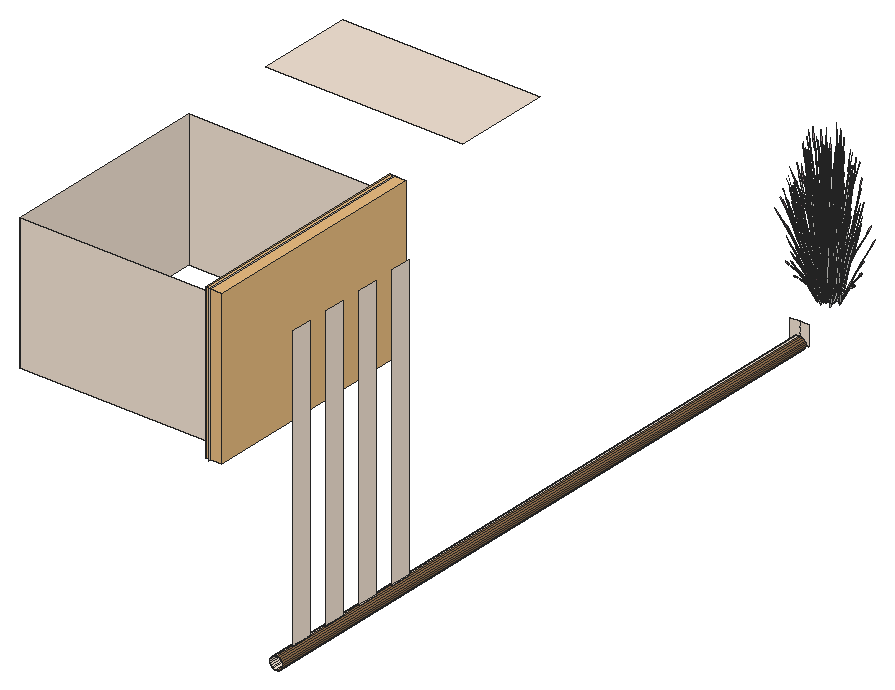
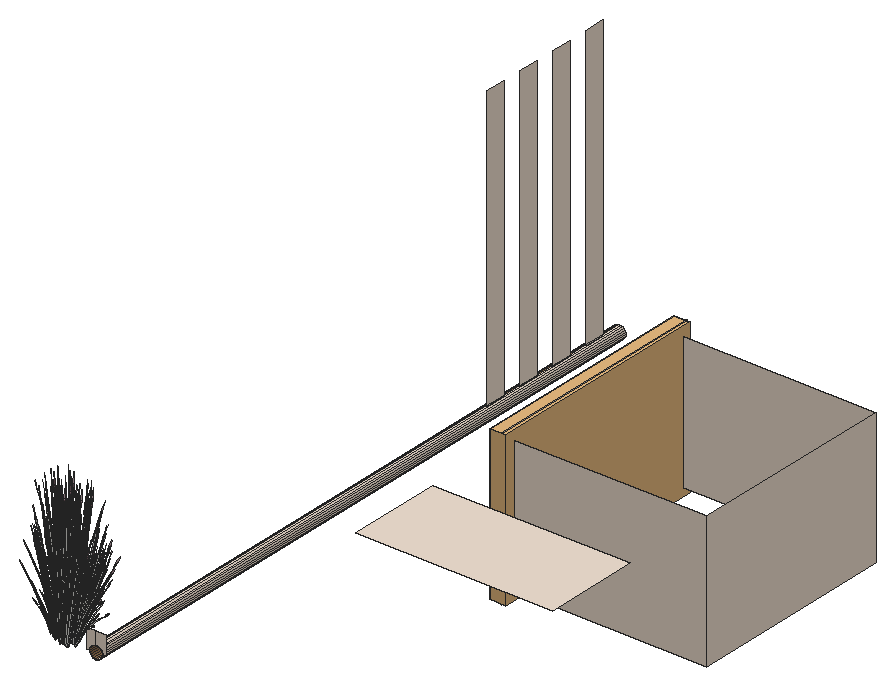
# SketchUp Ruby script. Lengths in inches.
U = 1.inch
M = Sketchup.active_model
def pt(a) = Geom::Point3d.new(a.map { |v| v * U })
def face(e, loops, mat)
  f = e.add_face(loops[0].map { |a| pt(a) })
  loops[1..].each { |l| e.add_face(l.map { |a| pt(a) }).erase! }
  f.material = f.back_material = mat if mat
  f
end
# faces: each face lists its corners as indices into pts; further lists are holes
def faces(e, pts, list, mat = nil) = list.each { |f| face(e, (f[0].is_a?(Array) ? f : [f]).map { |l| l.map { |i| pts[i] } }, mat) }
# xy, xz, yz: faces in a plane at the given z, y or x. An outline is a flat list of corners, or four numbers for a rectangle; further outlines are holes
def ring(l) = l.size == 4 ? [[l[0], l[1]], [l[2], l[1]], [l[2], l[3]], [l[0], l[3]]] : l.each_slice(2).to_a
def flat(e, list, mat, &to3) = list.each { |f| face(e, (f[0].is_a?(Array) ? f : [f]).map { |l| ring(l).map { |u, v| to3.(u, v) } }, mat) }
def xy(e, z, list, mat = nil) = flat(e, list, mat) { |x, y| [x, y, z] }
def xz(e, y, list, mat = nil) = flat(e, list, mat) { |x, z| [x, y, z] }
def yz(e, x, list, mat = nil) = flat(e, list, mat) { |y, z| [x, y, z] }
def lines(e, pts, list) = list.each { |a, b| e.add_line(pt(pts[a]), pt(pts[b])) }
# prism: a flat outline (further loops are holes) pulled along v
def prism(e, loops, v, mat = nil)
  f = face(e, loops, mat); d = Geom::Vector3d.new(v.map { |x| x * U })
  f.pushpull(f.normal.samedirection?(d) ? d.length : -d.length)
end
def box(e, o, s, mat = nil) = prism(e, [[o, [o[0] + s[0], o[1], o[2]], [o[0] + s[0], o[1] + s[1], o[2]], [o[0], o[1] + s[1], o[2]]]], [0, 0, s[2]], mat)
def at(x, y, z, deg = 0) = Geom::Transformation.translation(pt([x, y, z])) * Geom::Transformation.rotation(ORIGIN, Z_AXIS, deg.degrees)
def axes(o, x, y, z) = Geom::Transformation.new([*x, 0, *y, 0, *z, 0, *pt(o).to_a, 1])
def part(name) = M.definitions.add(name)
# library, detail: a bought-in or finely detailed component or shape, given as its bounding box
def library(name, o, s) = part(name).tap { |d| box(d.entities, o, s) }
def detail(e, o, s) = box(e.add_group.entities, o, s)
def put(e, d, t, mat = nil) = e.add_instance(d, t).tap { |i| i.material = mat if mat }
def group(e, t, mat = nil) = e.add_group.tap { |g| g.transformation = t; g.material = mat if mat }.entities
root = M.entities
M.materials.add("C01_Vanilla_Cream").color = [244, 228, 212]
M.materials.add("LightPink_Translucent").color = [144, 107, 117]
M.materials["LightPink_Translucent"].alpha = 0.75
M.materials.add("Wood_Floor_01_1K").color = [146, 111, 76]
c1 = library("Double casement window",[0,0,0],[5.02,56.42,60])
c2 = part("blade")
p = [[2.15,0.21,22],[0,0.17,0],[0.09,0.45,0],[2.18,0.31,22],[2.29,0.31,22],[0.38,0.45,0],
  [2.48,0.24,33],[2.49,0.24,33],[2.48,0.22,33]]
faces(c2.entities,p,[[0,1,2,3],[4,5,2,3],[6,3,4,7],[8,0,3,6]])
c3 = part("seeds")
p = [[0.3,-0.1,1.38],[-0.01,-0.03,1.59],[-0.01,-0.03,0.03],[0.14,-0.07,-0.07],[0.29,-0.03,3],[0.15,0.01,3.11]]
faces(c3.entities,p,[[0,1,2,3],[1,0,4,5]],"LightPink_Translucent")
c4 = part("blade with seeds")
put(c4.entities,c2,at(0,0,0))
put(c4.entities,c3,axes([2.4,0.25,30.99],[1.5799,-0.05474,1.17369],[-0.12525,1.92788,0.29478],[-0.07173,-0.02425,1.56792]))
xy(root,243,[[226.53,171,288,201]],"C01_Vanilla_Cream")
xz(root,75,[[226.53,201,288,243]],"C01_Vanilla_Cream")
xz(root,141,[[226.53,201,288,243]],"C01_Vanilla_Cream")
xz(root,216,[[354,192,355,192,355.07,192.52,355.27,193,355.59,193.41,356,193.73,356.48,193.93,357,194,357,198,354,198],[359,192,360,192,360,198,357,198,357,194,357.52,193.93,358,193.73,358.41,193.41,358.73,193,358.93,192.52]],"C01_Vanilla_Cream")
yz(root,226.53,[[75,201,141,243]],"C01_Vanilla_Cream")
yz(root,288,[[[72,198,144,246],[109.5,201,141,243],[75,201,106.5,243]]],"C01_Vanilla_Cream")
yz(root,357,[[18.46,190,24.91,194],[31.37,190,37.83,194],[44.28,190,50.74,194],[57.2,190,63.65,194],[18.46,194,24.91,282],
  [31.37,194,37.83,282],[44.28,194,50.74,282],[57.2,194,63.65,282]],"C01_Vanilla_Cream")
p = [[356.48,216,190.07],[357,216,190],[357,63.65,190],[357,57.2,190],[357,50.74,190],[357,44.28,190],
  [357,37.83,190],[357,31.37,190],[357,24.91,190],[357,18.46,190],[357,12,190],[356.48,12,190.07],
  [357.52,216,190.07],[357.52,12,190.07],[356,216,190.27],[356,12,190.27],[358,216,190.27],[358,12,190.27],
  [355.59,216,190.59],[355.59,12,190.59],[358.41,216,190.59],[358.41,12,190.59],[355.27,216,191],[355.27,12,191],
  [358.73,216,191],[358.73,12,191],[355.07,216,191.48],[355.07,12,191.48],[358.93,216,191.48],[358.93,12,191.48],
  [355,216,192],[355,12,192],[359,216,192],[359,12,192],[355.07,216,192.52],[355.07,12,192.52],
  [358.93,216,192.52],[358.93,12,192.52],[355.27,216,193],[355.27,12,193],[358.73,216,193],[358.73,12,193],
  [355.59,216,193.41],[355.59,12,193.41],[358.41,216,193.41],[358.41,12,193.41],[356,216,193.73],[356,12,193.73],
  [358,216,193.73],[358,12,193.73],[356.48,216,193.93],[356.48,12,193.93],[357.52,216,193.93],[357.52,12,193.93],
  [357,216,194],[357,12,194],[357,18.46,194],[357,24.91,194],[357,31.37,194],[357,37.83,194],
  [357,44.28,194],[357,50.74,194],[357,57.2,194],[357,63.65,194]]
faces(root,p,[[0,1,2,3,4,5,6,7,8,9,10,11],[14,0,11,15],[18,14,15,19],[22,18,19,23],[26,22,23,27],[30,26,27,31],[34,30,31,35],[38,34,35,39],
  [42,38,39,43],[46,42,43,47],[50,46,47,51],[54,50,51,55,56,57,58,59,60,61,62,63]],"C01_Vanilla_Cream")
faces(root,p,[[1,12,13,10,9,8,7,6,5,4,3,2],[12,16,17,13],[16,20,21,17],[20,24,25,21],[24,28,29,25],[28,32,33,29],[32,36,37,33],[36,40,41,37],
  [40,44,45,41],[44,48,49,45],[48,52,53,49],[52,54,63,62,61,60,59,58,57,56,55,53]],"Wood_Floor_01_1K")
put(root,c1,axes([286.7,72.24,198.3],[1,0,0],[0,1.27666,0],[0,0,0.79394]))
put(root,c4,axes([356.25,225,200.91],[0.12726,0.15818,1.28532],[-0.58807,0.13317,0.10393],[-0.13291,-0.24832,0.54946]))
put(root,c4,axes([357.22,223.95,201.54],[-0.08515,-0.06907,1.31208],[-0.56828,0.04379,-0.2075],[-0.0907,-0.16522,0.10523]))
put(root,c4,axes([358.54,224.77,199.94],[-0.15825,0.09972,1.07251],[-0.47395,-0.17454,-0.23066],[0.08785,-0.21706,0.45856]))
put(root,c4,axes([357.82,225.12,201.74],[-0.26572,-0.40059,-0.53284],[0.54698,-0.22325,0.0643],[-0.06214,-0.19355,0.75375]))
put(root,c4,axes([356.09,224.58,199.94],[-0.03371,0.16116,1.07251],[-0.49286,0.13491,-0.23066],[-0.11521,-0.20831,0.45856]))
put(root,c4,axes([357.36,224.23,199.12],[-0.09338,0.01775,1.32257],[-0.51641,-0.1998,-0.20205],[0.00867,-0.16666,0.22528]))
put(root,c4,axes([358.92,225.51,201.74],[0.01449,-0.45571,-0.53284],[0.61002,0.03061,0.0643],[0.06438,-0.19306,0.75375]))
put(root,c4,axes([359.77,224.8,201.54],[-0.00537,-0.09805,1.31208],[-0.45391,-0.28338,-0.2075],[0.07018,-0.17178,0.10523]))
put(root,c4,axes([357.87,224.78,201.39],[0.16784,-0.37886,-0.2656],[0.48968,0.1105,0.3429],[-0.0449,-0.15254,0.65611]))
put(root,c4,axes([358.24,225.28,200.91],[-0.10366,0.16934,1.28532],[-0.43488,-0.35044,0.10393],[0.19618,-0.21841,0.54946]))
put(root,c4,axes([359.65,224.44,201.53],[-0.05654,0.03763,1.33037],[-0.55396,-0.12696,-0.12571],[-0.02005,-0.16422,0.23543]))
put(root,c4,axes([357.62,225.04,201.51],[-0.54728,-0.1235,-0.38324],[0.18759,-0.42344,-0.29685],[-0.05018,-0.17048,0.7333]))
put(root,c4,axes([357.95,223.98,200.07],[0.07142,0.28728,0.86145],[-0.3962,-0.15911,0.63294],[0.04263,-0.1471,0.18974]))
put(root,c4,axes([358.8,225.36,201.51],[-0.39855,-0.33102,-0.38324],[0.42102,-0.2899,-0.29685],[0.06064,-0.16819,0.7333]))
put(root,c4,axes([356.64,223.72,201.53],[-0.01039,0.05905,1.33037],[-0.51226,0.21431,-0.12571],[-0.15074,-0.10955,0.23543]))
put(root,c4,axes([356.52,224.77,201.82],[0.62019,-0.12663,0.40322],[0.10763,0.49673,0.33247],[-0.14586,-0.1464,0.83437]))
put(root,c4,axes([357.93,224.86,201.55],[0.54859,0.1288,0.36002],[-0.18759,0.42344,0.29685],[-0.03297,-0.16652,0.74497]))
put(root,c4,axes([358.08,225.02,201.78],[-0.54481,0.22937,-0.0912],[-0.26773,-0.4071,-0.50621],[-0.07188,-0.17155,0.76918]))
put(root,c4,axes([359.22,225.53,201.78],[-0.61188,-0.02441,-0.0912],[0.01672,-0.46217,-0.50621],[0.0425,-0.178,0.76918]))
put(root,c4,axes([359.17,225.23,201.39],[0.3767,-0.25939,-0.2656],[0.3566,0.29618,0.3429],[0.05426,-0.15048,0.65611]))
put(root,c4,axes([355.92,224.32,200.07],[0.29042,0.17147,0.86145],[-0.42295,0.10307,0.63294],[-0.0905,-0.13178,0.18974]))
put(root,c4,axes([358.07,224.83,201.55],[0.41024,-0.16744,0.04823],[0.2008,0.30532,0.37966],[-0.03962,-0.13459,0.57892]))
put(root,c4,axes([356.62,225.23,201.74],[-0.47473,-0.23813,-0.53284],[0.33738,-0.41728,0.0643],[-0.172,-0.14218,0.75375]))
put(root,c4,axes([356.45,224.91,201.39],[-0.08599,-0.39682,-0.2656],[0.49155,-0.10478,0.3429],[-0.13203,-0.11372,0.65611]))
put(root,c4,axes([356.67,224.88,201.55],[0.25304,-0.31296,0.04823],[0.36033,0.18221,0.37966],[-0.11649,-0.10034,0.57892]))
put(root,c4,axes([355.6875,224.84,199.12],[-0.05393,0.0649,1.32257],[-0.545,0.13993,-0.20205],[-0.13166,-0.12729,0.22528]))
put(root,c4,axes([356.59,226.62,199.57],[-0.22864,-0.5052,-0.52377],[0.65862,-0.18195,-0.13747],[-0.02527,-0.17107,1.15612]))
put(root,c4,axes([355.4,225.49,200.91],[0.2068,0.08488,1.28532],[-0.42797,0.35609,0.10393],[-0.26673,-0.16064,0.54946]))
put(root,c4,axes([359.64,225.08,199.12],[-0.08333,-0.03881,1.32257],[-0.21404,-0.4336,-0.20205],[0.14439,-0.11767,0.22528]))
put(root,c4,axes([357.92,225.17,201.79],[-0.16784,0.37886,0.2656],[-0.48968,-0.1105,-0.3429],[-0.0449,-0.15254,0.65611]))
put(root,c4,axes([356.4,225.24,201.51],[-0.54938,0.11711,-0.38324],[-0.0961,-0.44351,-0.29685],[-0.14756,-0.1271,0.7333]))
put(root,c4,axes([359.17,225.33,201.55],[0.39645,0.33614,0.36002],[-0.42102,0.2899,0.29685],[0.07313,-0.15771,0.74497]))
put(root,c4,axes([356.78,224.85,202.07],[-0.37157,0.4723,-0.10215],[-0.5381,-0.2721,-0.56695],[-0.18705,-0.13344,0.86148]))
put(root,c4,axes([359.32,225.37,201.55],[0.45752,0.02296,0.04823],[-0.01254,0.34663,0.37966],[0.04787,-0.13278,0.57892]))
put(root,c4,axes([358.98,225.6,201.79],[-0.3767,0.25939,0.2656],[-0.3566,-0.29618,-0.3429],[0.05426,-0.15048,0.65611]))
put(root,c4,axes([359.64,226.3,201.74],[0.29081,-0.38873,-0.53284],[0.5096,0.27626,0.0643],[0.17364,-0.14084,0.75375]))
put(root,c4,axes([356.5,225.17,199.78],[-0.34808,-0.49367,0],[0.58235,-0.27531,-0.38706],[0.13264,-0.0627,1.22783]))
put(root,c4,axes([359.625,226.12,201.51],[-0.14302,-0.44985,-0.38324],[0.54163,-0.07869,-0.29685],[0.15522,-0.12083,0.7333]))
put(root,c4,axes([357.26,224.57,199.6],[-0.38473,0.28263,-0.02919],[-0.35252,-0.30954,-0.13237],[-0.02482,-0.08771,0.43661]))
put(root,c4,axes([355.36,224.71,201.54],[-0.11979,-0.00348,1.31208],[-0.38137,0.34775,-0.2075],[-0.20349,-0.07106,0.10523]))
put(root,c4,axes([359.88,226.44,201.78],[-0.515,-0.27165,-0.0912],[0.2967,-0.3934,-0.50621],[0.1455,-0.13675,0.76918]))
put(root,c4,axes([357.75,227.92,200.49],[0.48111,0.19866,1.13446],[-0.47133,0.42798,0.44862],[-0.21112,-0.25366,0.95105]))
put(root,c4,axes([356.75,225.24,201.79],[0.08599,0.39682,0.2656],[-0.49155,0.10478,-0.3429],[-0.13203,-0.11372,0.65611]))
put(root,c4,axes([355.24,226.55,199.51],[0,-0.49266,-0.37238],[0.62289,0,0],[0,-0.11221,1.18128]))
put(root,c4,axes([356.97,225.09,199.51],[0.52105,-0.24633,-0.37238],[0.31144,0.44171,0],[0.11867,-0.0561,1.18128]))
put(root,c4,axes([360.0625,225.94,199.94],[-0.19889,-0.01459,1.07251],[-0.20376,-0.39145,-0.23066],[0.24434,-0.11074,0.45856]))
put(root,c4,axes([355.27,225.5,201.82],[0.45978,-0.36358,0.40322],[0.39653,0.38611,0.33247],[-0.21571,-0.06707,0.83437]))
put(root,c4,axes([361.15,226.32,201.53],[-0.07272,-0.00374,1.33037],[-0.30197,-0.40092,-0.12571],[0.12127,-0.13182,0.23543]))
put(root,c4,axes([357.59,226.1,199.54],[0.375,-0.3703,-0.46765],[0.46584,0.33578,-0.12274],[0.15027,-0.09237,1.03225]))
put(root,c4,axes([360.29,225.22,200.07],[-0.18544,0.25079,0.86145],[-0.15939,-0.33694,0.63294],[0.15316,-0.08443,0.18974]))
put(root,c4,axes([360.03,226.17,201.39],[0.48462,-0.07041,-0.2656],[0.12797,0.4025,0.3429],[0.13888,-0.10811,0.65611]))
put(root,c4,axes([355.48,225.49,201.55],[0.02803,-0.37463,0.04823],[0.42332,0.01027,0.37966],[-0.16216,-0.0392,0.57892]))
put(root,c4,axes([356.93,226.75,199.66],[0.27012,-0.44393,-0.33554],[0.56127,0.21365,0.16149],[0,-0.10233,1.07733]))
put(root,c4,axes([355.32,225.61,201.39],[-0.31678,-0.30846,-0.2656],[0.36171,-0.29199,0.3429],[-0.18378,-0.04443,0.65611]))
put(root,c4,axes([357.18,226.53,200],[-0.06488,-0.56215,-0.21822],[0.6757,-0.03399,-0.37502],[0.11898,-0.07488,1.19781]))
put(root,c4,axes([355.51,226.5625,199.52],[0.38863,-0.30738,-0.23233],[0.38863,0.30738,0.23233],[0,-0.09901,1.0423]))
put(root,c4,axes([355.35,225.09,199.6],[-0.1606,0.40228,-0.02919],[-0.4943,-0.12375,-0.13237],[-0.07505,-0.0658,0.43661]))
put(root,c4,axes([359.63,226.4,201.79],[-0.48462,0.07041,0.2656],[-0.12797,-0.4025,-0.3429],[0.13888,-0.10811,0.65611]))
put(root,c4,axes([356.87,227.12,200],[-0.62699,-0.23507,-0.21822],[0.3019,-0.49615,-0.37502],[-0.0197,-0.12182,1.19781]))
put(root,c4,axes([355.08,226.92,199.78],[-0.69617,0,0],[0,-0.55062,-0.38706],[0,-0.12541,1.22783]))
put(root,c4,axes([355.2,225.94,199.94],[0.1087,0.13716,1.07251],[-0.25048,0.37284,-0.23066],[-0.25719,-0.08912,0.45856]))
put(root,c4,axes([357.09,225.29,199.52],[0.51941,0.1219,-0.23233],[-0.13078,0.42928,0.23233],[0.10471,-0.0495,1.0423]))
put(root,c4,axes([355.65,225.82,201.74],[-0.55654,-0.01186,-0.53284],[0.03738,-0.49951,0.0643],[-0.23578,-0.05271,0.75375]))
put(root,c4,axes([360.07,226.34,201.55],[0.3822,0.20719,0.04823],[-0.22252,0.29505,0.37966],[0.12254,-0.09539,0.57892]))
put(root,c4,axes([359.96,226.25,201.55],[0.13808,0.45342,0.36002],[-0.54163,0.07869,0.29685],[0.15963,-0.10664,0.74497]))
put(root,c4,axes([361.42,226.8,201.54],[0.07726,-0.07504,1.31208],[-0.09888,-0.46032,-0.2075],[0.19384,-0.08728,0.10523]))
put(root,c4,axes([355.625,226.78,199.75],[-0.51786,0.4142,0.23067],[-0.51817,-0.40984,-0.27369],[-0.01808,-0.11762,1.23664]))
put(root,c4,axes([354.9,225,201.53],[0.04127,0.04917,1.33037],[-0.19898,0.44196,-0.12571],[-0.20151,0.0032,0.23543]))
put(root,c4,axes([357.27,226.97,199.82],[0.6273,0.23878,0.18048],[-0.3019,0.49615,0.37502],[0,-0.11437,1.20407]))
put(root,c4,axes([357.03,227.64,199.83],[0.14756,-0.58378,-0.17572],[0.69966,0.10176,0.38453],[-0.12225,-0.08062,1.1733]))
put(root,c4,axes([355.47,225.92,201.51],[-0.40426,0.32635,-0.38324],[-0.35404,-0.34474,-0.29685],[-0.2054,-0.04965,0.7333]))
put(root,c4,axes([355.77,225.77,201.79],[0.31678,0.30846,0.2656],[-0.36171,0.29199,-0.3429],[-0.18378,-0.04443,0.65611]))
put(root,c4,axes([354.56,226.35,200.07],[0.35544,-0.03525,0.86145],[-0.22547,0.31061,0.63294],[-0.17565,-0.04659,0.18974]))
put(root,c4,axes([357.07,226.64,200.04],[-0.60457,0.03041,0.33554],[-0.05467,-0.50484,-0.16149],[0.10823,-0.05117,1.07733]))
put(root,c4,axes([355.68,225.58,201.78],[-0.02981,0.50103,-0.0912],[-0.56442,-0.01369,-0.50621],[-0.21738,-0.0348,0.76918]))
put(root,c4,axes([355.51,227.01,199.86],[0,0.49266,0.37238],[-0.62289,0,0],[0,-0.11221,1.18128]))
put(root,c4,axes([359.9,227.5,201.78],[-0.28012,-0.44611,-0.0912],[0.49717,-0.21923,-0.50621],[0.20951,-0.05886,0.76918]))
put(root,c4,axes([359.88,227.12,201.51],[0.15083,-0.44814,-0.38324],[0.51712,0.15361,-0.29685],[0.2082,-0.04109,0.7333]))
put(root,c4,axes([359.0625,225.29,199.78],[0.34808,-0.49367,0],[0.58235,0.27531,-0.38706],[0.13264,0.0627,1.22783]))
put(root,c4,axes([354.96,226.27,200.91],[0.23093,-0.01116,1.28532],[-0.15319,0.4836,0.10393],[-0.32909,-0.02991,0.54946]))
put(root,c4,axes([356.98,227.4,199.66],[-0.33445,-0.41351,-0.33554],[0.50659,-0.29119,0.16149],[-0.10823,-0.05117,1.07733]))
put(root,c4,axes([357.05,226.82,199.77],[0.24206,0.5509,0.34316],[-0.69162,0.19157,0.13466],[0.00845,-0.10123,1.19142]))
put(root,c4,axes([360.43,227.24,199.49],[-0.35858,0.05912,1.06187],[-0.05708,-0.47061,0.06078],[0.25115,-0.07123,0.60425]))
put(root,c4,axes([361.08,226.83,199.7],[-0.34516,-0.31503,-0.04866],[0.37803,-0.28865,-0.22062],[0.10711,-0.02032,0.72768]))
put(root,c4,axes([356.92,227.25,200.04],[-0.27012,0.44393,0.33554],[-0.56127,-0.21365,-0.16149],[0,-0.10233,1.07733]))
put(root,c4,axes([357.92,226.87,199.65],[0,-0.57005,0],[0.69617,0,0],[0,0,1.34592]))
put(root,c4,axes([358.76,225.55,199.86],[-0.52105,-0.24633,0.37238],[0.31144,-0.44171,0],[0.11867,0.0561,1.18128]))
put(root,c4,axes([359.78,227.28,201.74],[0.48922,-0.21758,-0.53284],[0.27264,0.44789,0.0643],[0.23638,-0.05088,0.75375]))
put(root,c4,axes([356.68,227.5625,199.54],[-0.57914,-0.08077,-0.46765],[0.12221,-0.49823,-0.12274],[-0.17283,-0.06037,1.03225]))
put(root,c4,axes([357.59,226.51,199.77],[-0.46162,0.4471,0.34316],[-0.54842,-0.39467,0.13466],[0.11129,-0.04462,1.19142]))
put(root,c4,axes([358.09,227.31,199.72],[-0.51786,-0.42404,-0.04598],[0.51817,-0.4243,0],[-0.01808,-0.01481,1.31678]))
put(root,c4,axes([356.79,225.77,199.86],[-0.16083,0.48962,0.13232],[-0.58854,-0.13856,0.26315],[0.10167,-0.00238,1.20305]))
put(root,c4,axes([359.71,227.37,201.79],[-0.46269,-0.13744,0.2656],[0.13495,-0.40096,-0.3429],[0.18628,-0.03677,0.65611]))
put(root,c4,axes([354.86,226.63,201.55],[0.15729,-0.44921,0.36002],[0.51712,0.15361,0.29685],[-0.20336,0.027,0.74497]))
put(root,c4,axes([356.54,226.17,199.2],[-0.548,0.19724,0.96696],[-0.17442,-0.56594,0.37572],[0.3365,0.00941,1.09981]))
put(root,c4,axes([358.01,226.32,199.96],[0.1074,-0.43968,0.1086],[0.52474,0.07632,-0.3101],[0.0955,0.04515,0.95058]))
put(root,c4,axes([354.83,226.51,201.55],[-0.20448,-0.33592,0.04823],[0.37288,-0.16442,0.37966],[-0.16437,0.03244,0.57892]))
put(root,c4,axes([357.11,227.36,199.77],[0.70367,0.1038,0.34316],[-0.1432,0.58624,0.13466],[-0.10283,-0.05661,1.19142]))
put(root,c4,axes([360.82,226.9375,199.12],[-0.0291,-0.0748,1.32257],[0.20181,-0.43752,-0.20205],[0.20357,-0.00629,0.22528]))
put(root,c4,axes([354.81,226.86,199.12],[0.01412,0.07764,1.32257],[-0.28464,0.40547,-0.20205],[-0.20218,-0.02044,0.22528]))
put(root,c4,axes([357.79,226.43,200.04],[-0.33445,-0.41351,0.33554],[0.50659,-0.29119,-0.16149],[0.10823,0.05117,1.07733]))
put(root,c4,axes([356.0625,228.32,199.52],[-0.13078,-0.42928,-0.23233],[0.51941,-0.1219,0.23233],[-0.10471,-0.0495,1.0423]))
put(root,c4,axes([356.73,228.3,199.86],[0.59825,-0.13076,0.13232],[0.14773,0.48663,0.26315],[-0.05336,-0.0709,1.20305]))
put(root,c4,axes([357.96,226.46,200],[0.56211,-0.32708,-0.21822],[0.3738,0.46216,-0.37502],[0.13869,0.04694,1.19781]))
put(root,c4,axes([360.2,227.32,201.39],[0.46269,0.13744,-0.2656],[-0.13495,0.40096,0.3429],[0.18628,-0.03677,0.65611]))
put(root,c4,axes([355.92,228.51,199.51],[-0.52105,-0.24633,-0.37238],[0.31144,-0.44171,0],[-0.11867,-0.0561,1.18128]))
put(root,c4,axes([359.38,225.59,199.51],[0.52105,0.24633,-0.37238],[-0.31144,0.44171,0],[0.11867,0.0561,1.18128]))
put(root,c4,axes([354.76,226.68,201.39],[-0.46269,-0.13744,-0.2656],[0.13495,-0.40096,0.3429],[-0.18628,0.03677,0.65611]))
put(root,c4,axes([358.39,227,199.65],[0.62289,0,0],[0,0.51004,0],[0,0,1.33805]))
put(root,c4,axes([357.33,227.64,200],[-0.56211,0.32708,-0.21822],[-0.3738,-0.46216,-0.37502],[-0.13869,-0.04694,1.19781]))
put(root,c4,axes([358.57,225.8,199.86],[-0.59825,0.13076,0.13232],[-0.14773,-0.48663,0.26315],[0.05336,0.0709,1.20305]))
put(root,c4,axes([358.93,226.83,200.91],[-0.23093,0.01116,1.28532],[0.15319,-0.4836,0.10393],[0.32909,0.02991,0.54946]))
put(root,c4,axes([359.23,225.77,199.52],[0.13078,0.42928,-0.23233],[-0.51941,0.1219,0.23233],[0.10471,0.0495,1.0423]))
put(root,c4,axes([360.13,227.49,201.55],[0.20448,0.33592,0.04823],[-0.37288,0.16442,0.37966],[0.16437,-0.03244,0.57892]))
put(root,c4,axes([358.1875,226.74,199.79],[-0.70367,-0.1038,0.36899],[0.1432,-0.58624,0.1448],[0.10283,0.05661,1.2811]))
put(root,c4,axes([360.09,227.37,201.55],[-0.15729,0.44921,0.36002],[-0.51712,-0.15361,0.29685],[0.20336,-0.027,0.74497]))
put(root,c4,axes([357.625,228.18,199.65],[-0.18165,-0.42474,0],[0.51872,-0.14874,0],[0,0,1.15778]))
put(root,c4,axes([357.28,227.78,199.96],[-0.1074,0.43968,0.1086],[-0.52474,-0.07632,-0.3101],[-0.0955,-0.04515,0.95058]))
put(root,c4,axes([355.24,226.64,201.79],[0.46269,0.13744,0.2656],[-0.13495,0.40096,-0.3429],[-0.18628,0.03677,0.65611]))
put(root,c4,axes([358.31,228.125,199.64],[0.5845,-0.16716,-0.14398],[0.20539,0.48152,0.00006],[0.06452,-0.01848,1.30423]))
put(root,c4,axes([358.51,228.32,199.86],[0.16083,-0.48962,0.13232],[0.58854,0.13856,0.26315],[-0.10167,0.00238,1.20305]))
put(root,c4,axes([358.375,227.21,199.66],[0.38863,0.31822,0],[-0.38863,0.31822,0],[0,0,1.2695]))
put(root,c4,axes([356.17,226.62,200.51],[0.15825,-0.07127,1.32798],[0.05457,0.4976,0.10393],[-0.34278,0.06603,0.47463]))
put(root,c4,axes([359.43,227.07,199.86],[-0.43742,-0.35886,0.13232],[0.44081,-0.34807,0.26315],[-0.04831,0.07329,1.20305]))
put(root,c4,axes([358.62,226.53,199.54],[0.57914,0.08077,-0.46765],[-0.12221,0.49823,-0.12274],[0.17283,0.06037,1.03225]))
put(root,c4,axes([361.18,227.4,200.07],[-0.34399,0.08133,0.86145],[0.16192,-0.33614,0.63294],[0.18249,0.023,0.18974]))
put(root,c4,axes([357.5,228.375,199.65],[-0.56127,-0.22118,0],[0.27012,-0.45959,0],[0,0,1.2203]))
put(root,c4,axes([357.96,227.79,199.85],[-0.54364,-0.39653,-0.18894],[0.45745,-0.44527,0.41347],[-0.14639,0.04639,1.26162]))
put(root,c4,axes([356.53,228.55,199.86],[0.52105,0.24633,0.37238],[-0.31144,0.44171,0],[-0.11867,-0.0561,1.18128]))
put(root,c4,axes([358.37,226.84,200.04],[0.27012,-0.44393,0.33554],[0.56127,0.21365,-0.16149],[0,0.10233,1.07733]))
put(root,c4,axes([361.02,228.83,201.53],[-0.05034,-0.04313,1.33037],[0.11012,-0.46232,-0.12571],[0.1983,-0.02954,0.23543]))
put(root,c4,axes([354.47,226.95,201.54],[-0.09091,0.06396,1.31208],[0.00773,0.46734,-0.2075],[-0.20839,0.06078,0.10523]))
put(root,c4,axes([358.27,227.1,199.72],[0,0.56976,-0.04228],[-0.69617,0,0],[0,0.01791,1.34526]))
put(root,c4,axes([355.07,226.89,201.51],[-0.15083,0.44814,-0.38324],[-0.51712,-0.15361,-0.29685],[-0.2082,0.04109,0.7333]))
put(root,c4,axes([355.05,226.5,201.78],[0.28012,0.44611,-0.0912],[-0.49717,0.21923,-0.50621],[-0.20951,0.05886,0.76918]))
put(root,c4,axes([358.32,226.69,199.66],[0.33445,0.41351,-0.33554],[-0.50659,0.29119,0.16149],[0.10823,0.05117,1.07733]))
put(root,c4,axes([360.58,228.44,200.95],[-0.10656,-0.41414,-0.02619],[0.50364,-0.09521,-0.11874],[0.10517,0.02626,0.39164]))
put(root,c4,axes([356.23,228.8,199.78],[-0.34808,0.49367,0],[-0.58235,-0.27531,-0.38706],[-0.13264,-0.0627,1.22783]))
put(root,c4,axes([359.27,228.43,201.78],[0.02981,-0.50103,-0.0912],[0.56442,0.01369,-0.50621],[0.21738,0.0348,0.76918]))
put(root,c4,axes([359.79,227.09,199.86],[0,-0.49266,0.37238],[0.62289,0,0],[0,0.11221,1.18128]))
put(root,c4,axes([358.23,227.46,200.04],[0.60457,-0.03041,0.33554],[0.05467,0.50484,-0.16149],[-0.10823,0.05117,1.07733]))
put(root,c4,axes([358.6,226.94,199.96],[0.51872,-0.14368,0.1086],[0.18165,0.41027,-0.3101],[0,0.09029,0.95058]))
put(root,c4,axes([359.1875,228.23,201.79],[-0.31678,-0.30846,0.2656],[0.36171,-0.29199,-0.3429],[0.18378,0.04443,0.65611]))
put(root,c4,axes([357.6875,227.7,199.66],[-0.60457,0.03041,-0.33554],[-0.05467,-0.50484,0.16149],[-0.10823,0.05117,1.07733]))
put(root,c4,axes([360.53,227.94,199.94],[-0.13408,-0.12117,1.07251],[0.17446,-0.40083,-0.23066],[0.27128,0.0543,0.45856]))
put(root,c4,axes([358.14,228.38,199.65],[0.56127,0.22118,0],[-0.27012,0.45959,0],[0,0,1.31215]))
